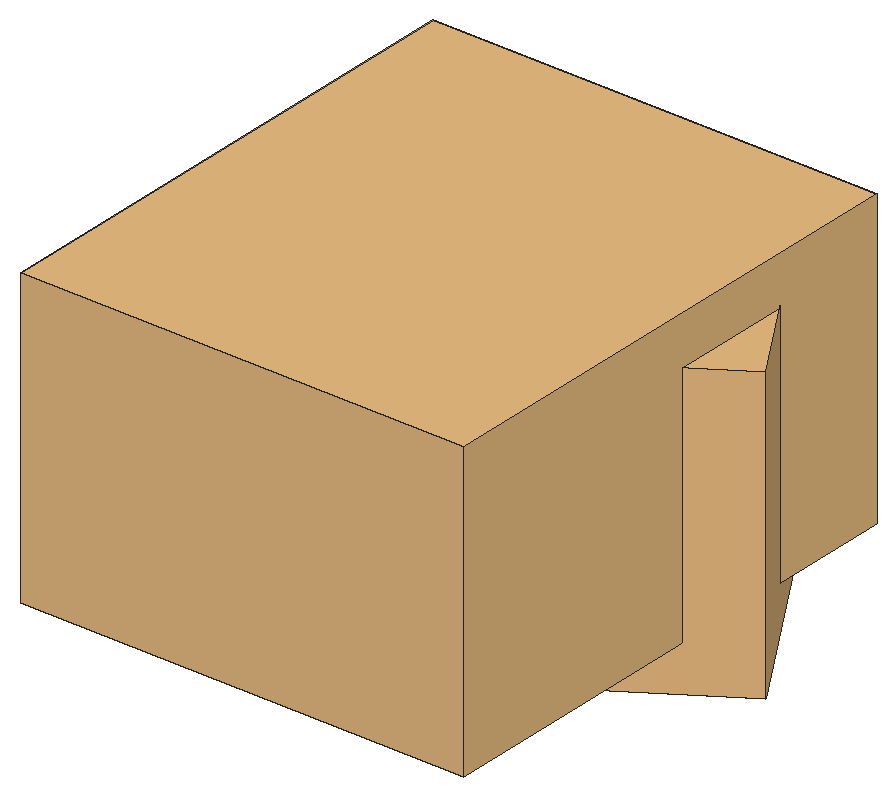
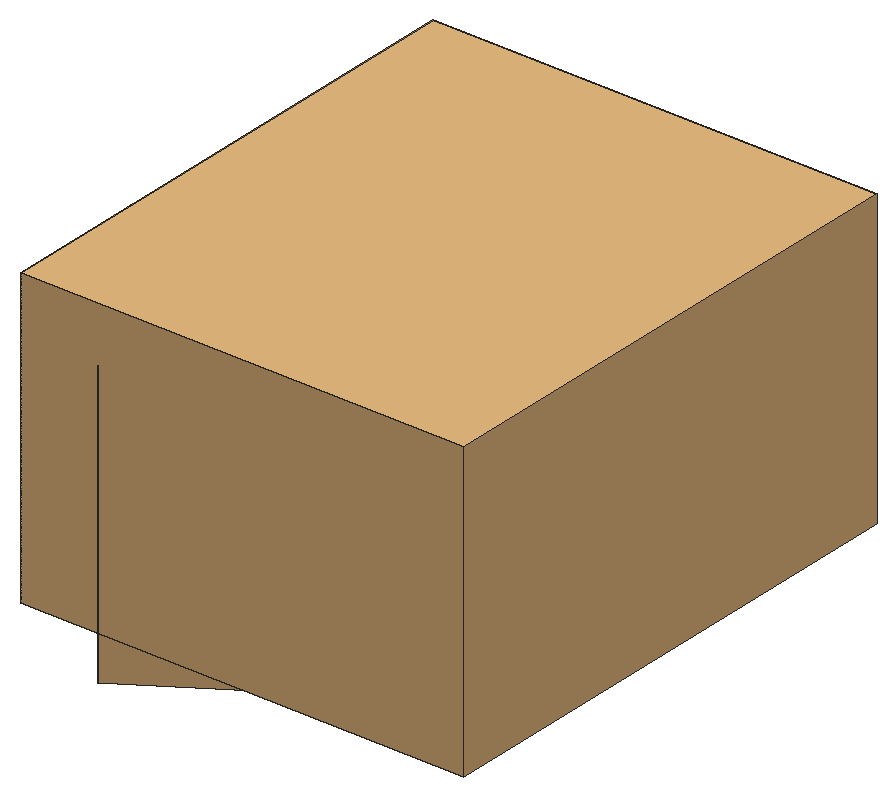
# SketchUp Ruby script. Lengths in inches.
U = 1.inch
M = Sketchup.active_model
def pt(a) = Geom::Point3d.new(a.map { |v| v * U })
def face(e, loops, mat)
  f = e.add_face(loops[0].map { |a| pt(a) })
  loops[1..].each { |l| e.add_face(l.map { |a| pt(a) }).erase! }
  f.material = f.back_material = mat if mat
  f
end
# faces: each face lists its corners as indices into pts; further lists are holes
def faces(e, pts, list, mat = nil) = list.each { |f| face(e, (f[0].is_a?(Array) ? f : [f]).map { |l| l.map { |i| pts[i] } }, mat) }
# xy, xz, yz: faces in a plane at the given z, y or x. An outline is a flat list of corners, or four numbers for a rectangle; further outlines are holes
def ring(l) = l.size == 4 ? [[l[0], l[1]], [l[2], l[1]], [l[2], l[3]], [l[0], l[3]]] : l.each_slice(2).to_a
def flat(e, list, mat, &to3) = list.each { |f| face(e, (f[0].is_a?(Array) ? f : [f]).map { |l| ring(l).map { |u, v| to3.(u, v) } }, mat) }
def xy(e, z, list, mat = nil) = flat(e, list, mat) { |x, y| [x, y, z] }
def xz(e, y, list, mat = nil) = flat(e, list, mat) { |x, z| [x, y, z] }
def yz(e, x, list, mat = nil) = flat(e, list, mat) { |y, z| [x, y, z] }
def lines(e, pts, list) = list.each { |a, b| e.add_line(pt(pts[a]), pt(pts[b])) }
# prism: a flat outline (further loops are holes) pulled along v
def prism(e, loops, v, mat = nil)
  f = face(e, loops, mat); d = Geom::Vector3d.new(v.map { |x| x * U })
  f.pushpull(f.normal.samedirection?(d) ? d.length : -d.length)
end
def box(e, o, s, mat = nil) = prism(e, [[o, [o[0] + s[0], o[1], o[2]], [o[0] + s[0], o[1] + s[1], o[2]], [o[0], o[1] + s[1], o[2]]]], [0, 0, s[2]], mat)
def at(x, y, z, deg = 0) = Geom::Transformation.translation(pt([x, y, z])) * Geom::Transformation.rotation(ORIGIN, Z_AXIS, deg.degrees)
def axes(o, x, y, z) = Geom::Transformation.new([*x, 0, *y, 0, *z, 0, *pt(o).to_a, 1])
def part(name) = M.definitions.add(name)
# library, detail: a bought-in or finely detailed component or shape, given as its bounding box
def library(name, o, s) = part(name).tap { |d| box(d.entities, o, s) }
def detail(e, o, s) = box(e.add_group.entities, o, s)
def put(e, d, t, mat = nil) = e.add_instance(d, t).tap { |i| i.material = mat if mat }
def group(e, t, mat = nil) = e.add_group.tap { |g| g.transformation = t; g.material = mat if mat }.entities
root = M.entities
M.materials.add("0ad16as01f6asdLeafVar1sfd015as60f1as6").color = [231, 235, 211]
M.materials.add("asdfasdf0165f6asdLeafVar1sfd015as60f1as6").color = [231, 235, 211]
M.materials.add("dw_stemssadfasdfa0sdf1s01d6w1").color = [90, 97, 50]
M.materials.add("viburnumblaasdfas0df1w06d").color = [98, 102, 84]
M.materials.add("viburnumbladsadfasdfad0w122").color = [125, 129, 119]
c1 = part("Component\#315")
p = [[0.25,0,0],[2.05,0.01,0.35],[1.81,4.2,1.66],[0,4.19,1.3125]]
faces(c1.entities,p,[[0,1,2,3]],"viburnumbladsadfasdfad0w122")
c2 = part("viburnumblad2")
put(c2.entities,c1,axes([-19.23,-4.49,-32.18],[83.35428,0,0],[0,79.38502,0],[0,0,83.35428]))
c3 = part("Component\#314")
p = [[0.14,0,0],[2.58,0.05,0.25],[2.44,5.11,2.64],[0,5.05,2.39]]
faces(c3.entities,p,[[0,1,2,3]],"viburnumblaasdfas0df1w06d")
c4 = part("viburnumblad1\#2")
put(c4.entities,c3,axes([-37.25,6.23,19.31],[75.98784,0,0],[0,65.50676,0],[0,0,75.98784]))
c5 = part("vdw_leaf\#1")
p = [[0,0,0],[-2.77,1.61,2.32],[-4.3125,6.1,4.5],[-3.97,13.49,6.09],[-2.47,18.57,6.3],[-0.2,22.73,5.75],
  [2.54,19.66,6.85],[4.3,15.93,7.09],[5.03,7.6,5.43],[3.32,1.76,2.74]]
faces(c5.entities,p,[[0,1,2,3,4,5],[0,5,6,7,8,9]],"0ad16as01f6asdLeafVar1sfd015as60f1as6")
c6 = part("dw_branch_3\#2")
p = [[-10.06,-1.6,62.9],[-0.2,1.54,-0.01],[-10.43,1.54,62.72],[0.18,-1.6,0.17],[-23.75,-21.66,88.91],[-25.7,-20.3,89.55],
  [13.4,11.62,104.56],[13.33,13.52,104.47],[-49.25,-41.87,130.3125],[-50.33,-40.21,130.71],[-4.97,21.13,143.98],[35.61,27.99,178.64],
  [-5.09,23.64,143.96],[35.32,29.14,178.46],[-67.7,-55.38,181.06],[-68.34,-54.45,181.62],[-22.8125,33.9,200.59],[-22.94,35.79,200.41],
  [56.61,36.78,229.75],[56.29,38.09,229.57],[-70.63,-67.46,248.85],[-70.72,-66.33,249.5],[-25.05,43.32,240.75],[-24.98,44.26,240.57]]
faces(c6.entities,p,[[0,1,2],[0,3,1],[4,2,5],[4,0,2],[6,0,2],[6,2,7],[8,4,5],[8,5,9],
  [10,6,7],[11,6,7],[10,7,12],[11,7,13],[14,8,9],[14,9,15],[16,10,12],[16,12,17],
  [18,11,13],[18,13,19],[20,14,15],[20,15,21],[22,16,17],[22,17,23]],"dw_stemssadfasdfa0sdf1s01d6w1")
c7 = part("dw_branch3\#2")
put(c7.entities,c5,axes([-70.33,-63.58,233.32],[-1.00752,0.412,0.78596],[-0.24851,-1.22189,0.32195],[0.83141,0.09817,1.01433]))
put(c7.entities,c5,axes([-66.93,-54.91,182.82],[-0.84976,-0.98359,0.33619],[0.99572,-0.74889,0.32577],[-0.05223,0.46521,1.22907]))
put(c7.entities,c5,axes([-46.12,-39.49,126.35],[1.23843,0.5364,0.23552],[-0.56438,0.94474,0.81599],[0.15707,-0.83465,1.07498]))
put(c7.entities,c5,axes([13.0625,13.13,104.77],[-1.01271,0.69982,-0.26884],[-0.74268,-0.99813,0.19939],[-0.10222,0.31872,1.21473]))
put(c7.entities,c5,axes([-18.87,30.42,186.42],[0.36309,1.06515,-0.56675],[-1.14134,0.49515,0.19939],[0.39128,0.45593,1.10754]))
put(c7.entities,c5,axes([-3.2,4.15,75.77],[-1.04153,0.55414,0.44243],[-0.23365,-1.01045,0.71554],[0.6695,0.50943,0.93801]))
put(c7.entities,c5,axes([23.2,19.41,136.3],[-0.65687,-1.11295,-0.05714],[1.05857,-0.61429,-0.20411],[0.15163,-0.1536,1.24868]))
put(c7.entities,c5,axes([-25.57,35.48,201.32],[-0.64726,0.62827,0.87973],[-0.71635,-1.0172,0.19939],[0.80962,-0.39773,0.87973]))
put(c7.entities,c5,axes([-36.37,-32.14,110.35],[-0.80747,1.09962,0.12544],[-0.83333,-0.50188,-0.96467],[-0.72833,-0.64487,0.96467]))
put(c7.entities,c5,axes([-9.89,26.72,156.79],[0.45529,1.02969,0.56572],[-1.16919,0.33753,0.32662],[0.11537,-0.64297,1.07744]))
put(c7.entities,c5,axes([-26.57,46.1,241.0625],[0.00015,0.80921,0.22536],[-0.83985,0.00446,-0.01542],[-0.01605,-0.22532,0.80906]))
put(c7.entities,c5,axes([-9.2,-2.58,61.06],[-1.10001,-0.40312,0.39014],[0.40883,-1.1116,0.00411],[0.35732,0.13566,1.14763]))
put(c7.entities,c5,axes([-69.91,-63.11,233.93],[1.36249,-0.1432,0],[0.13201,1.25603,0.5309],[-0.05549,-0.52799,1.26295]))
put(c7.entities,c5,axes([32.2,25.46,166.13],[0.06878,-1.29051,-0.05714],[1.22165,0.07415,-0.20411],[0.2113,-0.04403,1.24868]))
put(c7.entities,c5,axes([-5.68,-0.66,44.43],[-0.48448,-1.12287,0.17078],[0.98138,-0.33653,0.57135],[-0.48308,0.36756,1.04626]))
put(c7.entities,c5,axes([43.45,32.81,198.64],[0.5408,1.19584,0.14106],[-0.94242,0.32409,0.86557],[0.74952,-0.45533,0.98656]))
put(c7.entities,c5,axes([12.52,14.14,104.98],[1.02694,0.54888,0.41092],[-0.53566,1.05407,-0.06927],[-0.38969,-0.12321,1.13846]))
put(c7.entities,c5,axes([44.55,32.375,198.73],[-0.65687,-1.11295,-0.05714],[1.05857,-0.61429,-0.20411],[0.15163,-0.1536,1.24868]))
put(c7.entities,c5,axes([-5.67,21.17,141.44],[-1.10726,0.43603,-0.32953],[-0.49537,-1.03435,0.29588],[-0.17521,0.40597,1.12589]))
put(c7.entities,c5,axes([55.69,37.84,229.48],[0.18984,0.96334,0.18958],[-0.71996,0.0053,0.69399],[0.66755,-0.26823,0.69457]))
put(c7.entities,c5,axes([-21.52,36.85,205.2],[0.72606,-0.98817,0.14519],[0.94364,0.7084,0.10251],[-0.16885,0.05176,1.19664]))
put(c7.entities,c5,axes([-68.51,-56.35,196.07],[1.16319,0.72381,0],[-0.66725,1.0723,0.5309],[0.28049,-0.45075,1.26295]))
put(c7.entities,c6,at(0.01,-0.09,-0.02),"dw_stemssadfasdfa0sdf1s01d6w1")
put(c7.entities,c5,axes([-2.49,5.18,75.91],[0.78614,-0.90346,-0.30078],[0.86953,0.79562,-0.11715],[0.28546,-0.14014,1.16705]))
put(c7.entities,c5,axes([-23.125,-16.22,82.25],[0.32175,1.32576,0.12544],[-1.33153,0.31835,0.05068],[0.01989,-0.13382,1.3633]))
put(c7.entities,c5,axes([-23.75,41.99,230.3],[0.85958,-0.87451,0.14519],[0.66531,0.75721,0.62192],[-0.54076,-0.36226,1.01955]))
put(c7.entities,c5,axes([27.07,22.48,149.34],[0.92952,-0.64745,-0.62467],[0.50188,1.074,-0.36637],[0.71693,0.02135,1.04468]))
put(c7.entities,c5,axes([17.66,16.25,119.93],[-0.91649,0.83891,-0.3601],[-0.87434,-0.77966,0.40896],[0.0492,0.54447,1.14321]))
put(c7.entities,c5,axes([-68.37,-54.54,181.63],[0.32047,1.28399,0.35434],[-1.33153,0.31835,0.05068],[-0.03484,-0.35624,1.32241]))
put(c7.entities,c5,axes([-28.98,-27.1,96.48],[-0.8814,-0.35966,-0.98523],[0.75246,-1.11336,-0.26672],[-0.73065,-0.71272,0.91382]))
put(c7.entities,c5,axes([-15.23,28.43,172.72],[-1.21149,0.11898,0.32517],[-0.09739,-1.25259,0.09551],[0.33228,0.0667,1.21356]))
put(c7.entities,c5,axes([-17.5625,31.23,186.85],[-0.49275,-1.12287,0.14519],[0.95014,-0.33653,0.62192],[-0.53717,0.36756,1.01955]))
put(c7.entities,c5,axes([26.7,21.22,149.39],[-1.00104,0.22334,0.83093],[0.36894,-1.0402,0.72406],[0.77731,0.78134,0.72643]))
put(c7.entities,c5,axes([-31.125,-24.87,97.38],[0.75482,-0.86936,0.69068],[-0.00159,0.80023,1.00899],[-1.08766,-0.58016,0.45842]))
put(c7.entities,c5,axes([-71.21,-66.73,248.67],[0.25207,0.96771,0],[-0.8921,0.23237,0.38752],[0.375,-0.09768,0.92186]))
put(c7.entities,c5,axes([-24.11,41.05,229.55],[-1.11612,0.51924,-0.26884],[-0.56394,-1.10897,0.19939],[-0.15444,0.29694,1.21473]))
put(c7.entities,c5,axes([6.75,8.37,91.63],[-0.33418,-1.12287,0.39014],[1.13558,-0.33653,0.00411],[0.10478,0.36756,1.14763]))
put(c7.entities,c5,axes([-26,45.89,241.63],[-0.26986,-0.70824,-0.32129],[0.56818,-0.39091,0.38449],[-0.49365,-0.09775,0.63011]))
put(c7.entities,c5,axes([3.74,17.32,124.35],[0.22441,1.22913,-0.16274],[-1.07812,0.11178,-0.64246],[-0.61228,0.25367,1.07162]))
put(c7.entities,c5,axes([-5.44,22.27,140.88],[1.2203,0.00475,0.31374],[-0.097,1.20386,0.35905],[-0.29841,-0.37189,1.1663]))
put(c7.entities,c5,axes([-13.79,29.35,173.31],[0.83169,-0.90108,0.14519],[0.68877,0.73594,0.62192],[-0.55187,-0.34509,1.01955]))
put(c7.entities,c5,axes([-16.92,-7.26,72.98],[1.30647,0.30378,-0.27886],[0.07026,0.74892,1.14503],[0.40633,-1.10623,0.69861]))
put(c7.entities,c5,axes([4.8,17.55,125.22],[-0.25598,-1.17842,0.26559],[1.01553,-0.08455,0.60363],[-0.56975,0.35087,1.00767]))
put(c7.entities,c5,axes([5.3125,8.35,91.45],[0.00638,1.22913,-0.27714],[-1.16413,0.11178,0.46895],[0.48205,0.25367,1.13617]))
put(c7.entities,c5,axes([38.12,30.57,183.07],[1.12534,0.26182,-0.63833],[-0.46674,1.18829,-0.33545],[0.5081,0.51169,1.10563]))
put(c7.entities,c5,axes([-70.41,-60.38,214.47],[-0.41425,1.30587,0],[-1.20383,-0.38188,0.5309],[0.50605,0.16053,1.26295]))
put(c7.entities,c5,axes([37.03,28.75,180.67],[-1.12533,0.00102,-0.63799],[-0.00113,-1.2408,0],[-0.62497,0.00057,1.10237]))
put(c7.entities,c5,axes([30.71,25.35,165.96],[-0.1364,1.29314,0.22715],[-1.08768,-0.23921,0.70862],[0.73536,-0.11394,1.09026]))
put(c7.entities,c5,axes([-38.05,-30.84,110.67],[-0.31533,-1.27379,-0.2839],[1.018,-0.40311,0.67794],[-0.74394,-0.05723,1.08307]))
put(c7.entities,c5,axes([50.11,34.45,213.36],[-1.05669,0.74401,-0.05714],[-0.616,-0.82138,0.69675],[0.37221,0.60904,1.04705]))
put(c7.entities,c5,axes([-65.32,-58.78,200.07],[-1.14597,-0.19668,-0.6713],[0.21784,-1.26924,0],[-0.64812,-0.11124,1.139]))
put(c7.entities,c5,axes([-53.2,-43.37,143.59],[-0.72817,-1.09167,-0.2839],[0.82127,-0.72411,0.67794],[-0.71934,0.19815,1.08307]))
put(c7.entities,c5,axes([-61.1,-50.25,163.67],[-0.52887,1.19686,-0.30066],[-1.10762,-0.57104,-0.32484],[-0.42634,0.12264,1.23812]))
put(c7.entities,c5,axes([-54.12,-42.96,142.67],[0.32175,1.32576,0.12544],[-1.33153,0.31835,0.05068],[0.01989,-0.13382,1.3633]))
put(c7.entities,c5,axes([22.03,20.08,132.3],[1.17066,0.5058,-0.34078],[-0.35758,1.16671,0.50333],[0.49407,-0.35407,1.17172]))
put(c7.entities,c5,axes([-8.59,26.04,158.21],[-0.49275,-1.12287,0.14519],[0.95014,-0.33653,0.62192],[-0.53717,0.36756,1.01955]))
put(c7.entities,c5,axes([49.92,34.03,213.7],[1.24742,-0.35176,0.25024],[0.42127,1.159,-0.4708],[-0.09426,0.52477,1.20753]))
put(c7.entities,c5,axes([-70.34,-67.02,249.05],[-0.57048,-0.79684,0],[0.73827,-0.52855,0.24329],[-0.20203,0.14464,0.92729]))
put(c7.entities,c5,axes([56.04,36.81,228.63],[0.33451,-0.90845,-0.15237],[0.87636,0.33365,-0.06538],[0.11487,-0.11636,0.94597]))
put(c7.entities,c5,axes([-69.93,-60.58,214.88],[-0.45293,-0.99272,-0.78227],[1.14635,-0.58199,0.07483],[-0.40282,-0.65636,1.06615]))
put(c7.entities,c5,axes([-16.77,-8.59,72.7],[-1.22785,0.11509,0.53076],[-0.24879,-1.22495,-0.30991],[0.46742,-0.38989,1.16587]))
put(c7.entities,c5,axes([18.29,17.18,119.24],[1.19981,-0.45946,0.3029],[0.40159,1.22775,0.27158],[-0.37626,-0.1547,1.25575]))
put(c7.entities,c5,axes([-6.73,-0.68,43.74],[0.05346,1.22913,-0.27201],[-1.22696,0.11178,0.26396],[0.28163,0.25367,1.20164]))
put(c7.entities,c5,axes([-58.57,-48.42,160.98],[0.43385,-1.23789,0.39533],[1.04879,0.57965,0.66404],[-0.76727,0.09236,1.13122]))
put(c7.entities,c5,axes([-23.4,38.49,215.38],[0.06762,1.22913,-0.26884],[-1.23909,0.11178,0.19939],[0.21835,0.25367,1.21473]))
put(c7.entities,c5,axes([-22.21,-16.62,83.17],[-0.72817,-1.09167,-0.2839],[0.82127,-0.72411,0.67794],[-0.71934,0.19815,1.08307]))
put(c7.entities,c5,axes([-45.7,-40.77,126.53],[-1.33715,-0.0713,-0.0976],[0.07167,-1.28508,-0.04314],[-0.09306,-0.0492,1.31098]))
put(c7.entities,c5,axes([-22.39,38.51,216.12],[-0.49275,-1.12287,0.14519],[0.95014,-0.33653,0.62192],[-0.53717,0.36756,1.01955]))
c8 = part("vdw_leaf\#2")
p = [[0,0,0],[-2.77,1.61,2.32],[-4.3125,6.1,4.5],[-3.97,13.49,6.09],[-2.47,18.57,6.3],[-0.2,22.73,5.75],
  [2.54,19.66,6.85],[4.3,15.93,7.09],[5.03,7.6,5.43],[3.32,1.76,2.74]]
faces(c8.entities,p,[[0,1,2,3,4,5],[0,5,6,7,8,9]],"asdfasdf0165f6asdLeafVar1sfd015as60f1as6")
c9 = part("dg_branch_1\#2")
p = [[46.12,1.57,35.62],[46,5.42,35.41],[0.14,1.79,0.05],[0.26,-2.0625,0.27],[74.05,2.99,75.8],[74.11,5.28,75.58],
  [103.46,0.47,94.74],[104.03,2.92,94.84],[81.14,16.92,120.46],[81.2,18.78,120.24],[130.47,-5.6875,130.27],[130.58,-3.66,129.85],
  [80.82,34.4375,191.22],[80.64,35.93,190.9],[148.49,-14.56,203.24],[148.9,-12.8125,203.11],[81.08,37.95,226.93],[81.4,39.1,227.03],
  [157.45,-18.19,250.77],[157.7,-17.01,250.41]]
faces(c9.entities,p,[[0,1,2,3],[4,0,1],[4,1,5],[6,4,5],[6,5,7],[8,4,5],[8,5,9],[10,6,7],
  [10,7,11],[12,8,9],[12,9,13],[14,10,11],[14,11,15],[16,12,13],[16,13,17],[18,14,15],
  [18,15,19]],"dw_stemssadfasdfa0sdf1s01d6w1")
c10 = part("vdw_branch1\#3")
put(c10.entities,c8,axes([120.69,-2.42,117.31],[1.12221,-0.24063,-0.65809],[0.19207,1.24776,-0.12871],[0.65778,0.01392,1.11658]))
put(c10.entities,c8,axes([81,38.9,226.05],[0.7888,-0.58155,0],[0.48308,0.65523,0.47],[-0.28484,-0.38635,0.83138]))
put(c10.entities,c8,axes([78.08,12.69,106.05],[-1.43826,-0.02353,-0.03177],[0.0088,-1.31777,0.57755],[-0.03854,0.57714,1.31741]))
put(c10.entities,c8,axes([130.18,-4.73,130.41],[-0.38031,-1.29044,-0.11242],[1.20662,-0.31032,-0.51987],[0.47109,-0.24694,1.24081]))
put(c10.entities,c8,axes([157.08,-17.89,249.93],[-0.91355,0.40674,0],[-0.37496,-0.84216,0.38752],[0.15762,0.35401,0.92186]))
put(c10.entities,c8,axes([90.64,3.03,86.49],[0.32514,-0.85045,-0.99675],[0.69523,0.98247,-0.61148],[1.11061,-0.36604,0.67459]))
put(c10.entities,c8,axes([80.15,28.42,160.95],[-0.16039,0.95636,-1.06292],[-1.41646,0.03966,0.24943],[0.19509,1.07422,0.93709]))
put(c10.entities,c8,axes([126.74,-5.45,129.22],[-0.59819,0.96152,-0.6841],[-0.85772,0.12575,0.92675],[0.75427,0.88089,0.57856]))
put(c10.entities,c8,axes([133.22,-6.12,150.66],[-0.93823,0.76985,0.59124],[-0.47726,-1.08188,0.65135],[0.84525,0.24366,1.02405]))
put(c10.entities,c8,axes([80.43,22.89,141.32],[-1.42571,-0.19312,0.01373],[0.18338,-1.31425,0.5561],[-0.0621,0.5528,1.32692]))
put(c10.entities,c8,axes([33.14,0.88,26.42],[-0.13338,1.31536,0.04876],[-1.04528,-0.13221,0.7073],[0.72315,0.03348,1.07497]))
put(c10.entities,c8,axes([152.63,-15.08,221.76],[-1.28188,0.41945,0.0579],[-0.3638,-1.18547,0.53367],[0.21665,0.49113,1.23869]))
put(c10.entities,c8,axes([80.05,28.28,160.33],[-0.46732,-1.26661,0.40679],[1.27397,-0.40257,0.21004],[-0.07408,0.44645,1.30501]))
put(c10.entities,c8,axes([153.95,-14.8,235.875],[0.39005,1.07743,0.20605],[-0.96443,0.25296,0.50293],[0.42961,-0.3464,0.99807]))
put(c10.entities,c8,axes([80.2,24.22,141.74],[1.33062,-0.46576,0.02628],[0.44746,1.2746,-0.06608],[-0.00197,0.0722,1.37936]))
put(c10.entities,c8,axes([145.48,-12.5,188.92],[-1.32952,0.16983,0.16138],[-0.09299,-1.2361,0.53471],[0.21503,0.51548,1.22904]))
put(c10.entities,c8,axes([139.64,-9.18,171.24],[0.05682,1.30088,0.23414],[-1.13176,-0.05343,0.57151],[0.58357,-0.22963,1.13417]))
put(c10.entities,c8,axes([70.95,4.35,71.98],[-1.1081,-0.41873,0.64752],[0.33675,-1.28259,-0.25313],[0.6937,-0.04625,1.15721]))
put(c10.entities,c8,axes([59.85,4.55,56.17],[-0.26797,1.24526,0.35754],[-0.9369,-0.41634,0.74783],[0.83377,-0.10389,0.98674]))
put(c10.entities,c8,axes([33.11,3.36,25.66],[-0.57817,-1.07968,-0.5679],[1.11554,-0.21356,-0.7297],[0.49375,-0.78178,0.98363]))
put(c10.entities,c9,at(-0.21,0.34,-0.17),"dw_stemssadfasdfa0sdf1s01d6w1")
put(c10.entities,c8,axes([80.91,19.01,122.53],[-0.84258,1.13222,-0.27981],[-1.15093,-0.75138,0.42537],[0.18861,0.47293,1.3457]))
put(c10.entities,c8,axes([119.8,-1.22,114.1],[-1.3235,-0.25012,0.09101],[0.25933,-1.31572,0.15537],[0.05991,0.1698,1.33794]))
put(c10.entities,c8,axes([46.29,5.1,38.04],[0.98937,0.73827,-0.47585],[-0.72359,1.03721,0.10473],[0.44068,0.18581,1.20453]))
put(c10.entities,c8,axes([81.1875,33.03,184.45],[1.33883,0.26986,0.35053],[-0.09581,1.22087,-0.57399],[-0.42216,0.53228,1.20262]))
put(c10.entities,c8,axes([80.16,36.28,206.98],[-0.83993,0.85737,-0.6234],[-1.05964,-0.65701,0.5241],[0.02941,0.81391,1.07976]))
put(c10.entities,c8,axes([154.86,-16.15,234.87],[0.02509,-1.15302,-0.28506],[1.1487,-0.04894,0.29908],[-0.30202,-0.28195,1.11384]))
put(c10.entities,c8,axes([108.77,-0.33,101.14],[-0.47691,-1.03266,-0.72709],[1.25395,-0.29455,-0.40416],[0.15052,-0.81814,1.06325]))
put(c10.entities,c8,axes([89.79,3.01,85.87],[-0.61344,0.75518,0.8965],[-0.17758,-1.01824,0.73622],[1.13385,0.22574,0.58569]))
put(c10.entities,c8,axes([81.56,20.31,123.29],[0.37259,-1.3435,0.21057],[1.29385,0.32364,-0.22445],[0.16906,0.25791,1.34638]))
put(c10.entities,c8,axes([46.45,1.82,36.74],[-0.77883,0.29892,1.0614],[0.19124,-1.24314,0.49044],[1.08598,0.43329,0.67484]))
put(c10.entities,c8,axes([71.37,4.02,72.32],[0.72905,0.81546,-0.74421],[-0.66805,0.98958,0.42988],[0.8391,0.14186,0.97745]))
put(c10.entities,c8,axes([136.59,-5.88,150.53],[0.85845,-0.99897,-0.12437],[0.96526,0.81273,0.13453],[-0.02572,-0.18182,1.28292]))
put(c10.entities,c8,axes([80.375,38.8,225.86],[-0.25178,0.96778,0],[-0.89216,-0.23211,0.38752],[0.37503,0.09757,0.92186]))
put(c10.entities,c8,axes([74.43,7.99,85.38],[-1.05703,0.91669,-0.33543],[-0.95806,-0.87958,0.61531],[0.18697,0.6754,1.25659]))
put(c10.entities,c8,axes([76.57,9.74,89.32],[0.63146,-1.21538,0.33508],[1.18148,0.49387,-0.43517],[0.26321,0.48577,1.26593]))
put(c10.entities,c8,axes([81.6875,36.97,207.4],[0.09422,-1.04424,0.38486],[1.01646,0.1939,0.27727],[-0.33299,0.33382,0.98727]))
put(c10.entities,c8,axes([157.29,-17.17,249.98],[0.50586,-0.50586,0],[0.38853,0.38853,0.41105],[-0.29684,-0.29684,0.56115]))
put(c10.entities,c8,axes([79.92,15.8,106.09],[1.03917,-0.29343,-0.90675],[-0.14587,1.22131,-0.5624],[0.92163,0.5191,0.88824]))
put(c10.entities,c8,axes([61.95,3.88,56.26],[0.41243,-1.28546,0],[1.17466,0.37688,-0.54831],[0.5221,0.16751,1.23363]))
put(c10.entities,c8,axes([151.99,-14.79,208.15],[-0.48571,-1.21723,-0.32393],[1.25386,-0.50033,0],[-0.12005,-0.30087,1.31056]))
put(c10.entities,c8,axes([108.44,0.62,102.22],[0.82183,0.96078,0.38967],[-0.62327,0.08618,1.10203],[0.79141,-0.88661,0.51693]))
put(c10.entities,c8,axes([145.6,-10.56,188.62],[1.03241,-0.02554,-0.82693],[0.3944,1.11584,0.45794],[0.70325,-0.61672,0.89706]))
put(c10.entities,c8,axes([78.59,32.3,183.89],[-1.12675,-0.42036,0.43987],[0.5899,-0.98149,0.57312],[0.14901,0.70693,1.05726]))
put(c10.entities,c8,axes([152.08,-13.42,223.37],[0.79993,-0.44251,-0.69938],[0.68456,0.82615,0.26026],[0.41048,-0.60953,0.85515]))
put(c10.entities,c8,axes([140.71,-8.74,170.55],[0.41903,-1.24177,-0.32393],[1.26224,0.33728,0.33986],[-0.23168,-0.40836,1.26573]))
put(c10.entities,c8,axes([149.25,-12.53,205.78],[1.24456,0.38285,0.23414],[-0.42999,1.04826,0.57151],[-0.02056,-0.62679,1.13417]))
c11 = part("vdw_leaf\#3")
p = [[0,0,0],[-2.77,1.61,2.32],[-4.3125,6.1,4.5],[-3.97,13.49,6.09],[-2.47,18.57,6.3],[-0.2,22.73,5.75],
  [2.54,19.66,6.85],[4.3,15.93,7.09],[5.03,7.6,5.43],[3.32,1.76,2.74]]
faces(c11.entities,p,[[0,1,2,3,4,5],[0,5,6,7,8,9]],"asdfasdf0165f6asdLeafVar1sfd015as60f1as6")
c12 = part("dw_brancj_2\#2")
p = [[9.7,-0.22,29.95],[0.23,-1.96,0.34],[-0.05,1.51,0.11],[9.65,1.51,29.46],[18.64,-8.75,84.43],[18.96,-6.63,84.625],
  [1.53,6.02,63.68],[1.42,8.18,63.25],[-10.58,8.77,161.17],[-10.41,9.98,160.68],[26.34,-9.37,211.72],[26.57,-8.28,211.23]]
faces(c12.entities,p,[[0,1,2],[0,2,3],[4,0,3],[4,3,5],[6,0,3],[6,3,7],[8,6,7],[8,7,9],
  [10,4,5],[10,5,11]],"dw_stemssadfasdfa0sdf1s01d6w1")
c13 = part("vdw_branch2\#3")
put(c13.entities,c11,axes([19.53,-5.9,102.42],[1.12377,-0.50004,0],[0.46097,1.03596,0.47664],[-0.19377,-0.43548,1.13389]))
put(c13.entities,c11,axes([-5.89,6.52,109.44],[-1.07209,0.83679,0],[-0.77141,-0.98832,0.52702],[0.32427,0.41545,1.25373]))
put(c13.entities,c11,axes([-0.44,8.23,75.28],[0.88709,-0.9947,0],[0.92159,0.82189,0.33087],[-0.25219,-0.22491,1.26111]))
put(c13.entities,c11,axes([24.71,-8.97,190.81],[-0.82641,0.91101,0],[-0.83983,-0.76184,0.47664],[0.35303,0.32025,1.13389]))
put(c13.entities,c11,axes([-2.29,8.24,91.35],[1.24603,-0.47303,0],[0.43826,1.15445,0.33087],[-0.11993,-0.31592,1.26111]))
put(c13.entities,c11,axes([12.26,-3.11,37.92],[-0.64625,1.02205,0.22511],[-1.04383,-0.61044,-0.22511],[-0.07533,-0.30931,1.18809]))
put(c13.entities,c11,axes([26.17,-9.17,210.27],[-0.99452,-0.10453,0],[0.09636,-0.91681,0.38752],[-0.04051,0.38539,0.92186]))
put(c13.entities,c11,axes([-6.07,9.4,125.35],[-0.90214,-0.98107,0],[0.90896,-0.83583,0.33087],[-0.24874,0.22873,1.26111]))
put(c13.entities,c11,axes([-4.13,7.29,110.58],[0.44715,-1.078,0.64369],[1.05816,0.63649,0.33087],[-0.58725,0.40856,1.09216]))
put(c13.entities,c11,axes([23.91,-8.22,171.96],[0.62307,0.85009,-0.63406],[-0.71531,0.8798,0.47664],[0.78296,0.12729,0.94004]))
put(c13.entities,c12,at(-0.09,0.18,-0.25),"dw_stemssadfasdfa0sdf1s01d6w1")
put(c13.entities,c11,axes([23.34,-9.65,156.59],[-0.31364,-1.00782,0.58216],[1.10369,-0.17062,0.29925],[-0.17137,0.6239,0.98776]))
put(c13.entities,c11,axes([15.03,-3.37,58.83],[-1.05425,-0.00194,0.58442],[-0.14303,-1.11707,-0.26172],[0.55355,-0.3046,0.99755]))
put(c13.entities,c11,axes([-11.625,9.46,160.37],[0.36812,0.92978,0],[-0.85713,0.33936,0.38752],[0.3603,-0.14265,0.92186]))
put(c13.entities,c11,axes([21.32,-8.53,138.72],[1.21379,0.19904,0],[-0.19904,1.21379,0],[0,0,1.23]))
put(c13.entities,c11,axes([22.54,-9.2,141.43],[-1.02887,0.17955,0.60182],[-0.23387,-1.13057,-0.06253],[0.56696,-0.17376,1.02111]))
put(c13.entities,c11,axes([23.9,-8.82,173.84],[-1.14567,-0.37474,0],[0.35918,-1.0981,0.04438],[-0.01409,0.04308,1.17993]))
put(c13.entities,c11,axes([-7.84,8.92,143.59],[-1.26971,0.40522,0],[-0.37543,-1.17638,0.33087],[0.10274,0.32192,1.26111]))
put(c13.entities,c11,axes([19.77,-8.01,85.98],[-0.32405,-1.14591,0.18674],[1.10278,-0.32969,-0.10948],[0.15845,0.14442,1.16117]))
put(c13.entities,c11,axes([-0.62,5.76,76.34],[-0.08879,1.17576,-0.67771],[-1.34525,-0.16582,-0.11144],[-0.17897,0.66309,1.17383]))
put(c13.entities,c11,axes([20.49,-8.22,121.07],[0.39924,-0.78471,-0.8233],[1.08735,0.33121,0.2116],[0.09035,-0.83005,0.83495]))
put(c13.entities,c11,axes([15.15,-3.72,62.9],[1.16251,0.40128,-0.0211],[-0.39924,1.16074,0.07874],[0.0456,-0.06757,1.2273]))
put(c13.entities,c11,axes([20.72,-8.08,120.26],[-0.03693,1.2277,-0.06551],[-1.22944,-0.03698,0],[-0.00197,0.06548,1.22825]))
put(c13.entities,c11,axes([22.58,-8.36,155.57],[-0.56247,1.09386,0],[-1.00839,-0.51852,0.47664],[0.42389,0.21796,1.13389]))
put(c13.entities,c11,axes([3.97,3.13,57.96],[-1.09459,0.76041,0],[-0.72262,-1.0402,-0.1735],[-0.10109,-0.14552,1.29352]))
put(c13.entities,c11,axes([-10.8,9.06,160.75],[-0.66334,-0.72138,0],[0.66835,-0.61458,0.24329],[-0.1829,0.16818,0.92729]))
put(c13.entities,c11,axes([19.06,-9.3125,103.96],[-1.01345,0.25553,-0.60051],[-0.2265,-1.12952,-0.09839],[-0.59598,0.03076,1.01889]))
put(c13.entities,c11,axes([18.07,-6.2,81.7],[-0.56247,1.09386,0],[-1.00839,-0.51852,0.47664],[0.42389,0.21796,1.13389]))
put(c13.entities,c11,axes([12.95,-0.39,43.31],[0.13044,-1.19832,0],[1.11025,0.12085,0.29925],[-0.30382,-0.03307,1.14057]))
put(c13.entities,c11,axes([2.28,8.28,56.18],[1.32413,-0.31027,0],[0.30923,1.31968,-0.11144],[0.02542,0.1085,1.35543]))
put(c13.entities,c11,axes([-7.55,9.96,143.07],[1.34251,-0.21744,0],[0.20045,1.23761,0.52702],[-0.08426,-0.52024,1.25373]))
put(c13.entities,c11,axes([26.15,-8.25,210.66],[0.94661,-0.25364,0],[0.235,0.87703,0.24329],[-0.06431,-0.24,0.92729]))
put(c13.entities,c11,axes([-6.48,11.37,125.16],[0.64635,1.10315,0.46356],[-1.16569,0.46153,0.52702],[0.27017,-0.6478,1.16488]))
put(c13.entities,c11,axes([25.74,-8.35,191.28],[0.13044,-1.19832,0],[1.11025,0.12085,0.29925],[-0.30382,-0.03307,1.14057]))
put(c13.entities,c11,axes([-5.125,7.47,91.6],[-1.10024,0.63688,0.48318],[-0.78682,-1.00808,-0.46292],[0.14137,-0.65404,1.184]))
c14 = library("Broadleaf plant",[0,0,0],[62.33,72.62,41.59])
c15 = library("Narrowleaf plant",[-0.44,-0.75,-1.28],[7.48,8.05,9.01])
put(root,c2,axes([2217.49,336.92,16.58],[-0.00784,0.00117,0.00859],[-0.00546,-0.0084,-0.00383],[0.00631,-0.00716,0.00674]))
put(root,c2,axes([2214.78,333.28,28.73],[0.00871,-0.00384,-0.00541],[0.00664,0.00406,0.00749],[-0.00079,-0.00912,0.00457]))
put(root,c2,axes([2214.99,335.42,27.42],[0.00909,-0.00401,-0.00564],[0.00597,0.00365,0.00674],[-0.00079,-0.00912,0.00457]))
put(root,c2,axes([2216.93,338.17,16.16],[-0.01071,-0.0052,0.00268],[0.00135,-0.00683,-0.00788],[0.0054,-0.00736,0.0073]))
put(root,c2,axes([2216.82,342,22.89],[-0.01242,-0.00411,0.00252],[0.00364,-0.01255,-0.00256],[0.00316,-0.0017,0.01283]))
put(root,c2,axes([2215.32,334.5625,28.24],[0.00143,-0.00635,-0.00868],[0.00992,-0.00012,0.00155],[-0.0013,-0.00861,0.00528]))
put(root,c4,axes([2216.48,338.3,27.22],[0.01164,0.00293,-0.00079],[-0.00215,0.01041,0.00877],[0.00216,-0.00738,0.00809]))
put(root,c2,axes([2216.16,333.26,28.67],[-0.00668,-0.00514,-0.00687],[0.00865,-0.00485,-0.0047],[-0.00103,-0.00803,0.00606]))
put(root,c2,axes([2216.17,335.37,27.46],[-0.00601,-0.0039,-0.00689],[0.00865,-0.00485,-0.0047],[-0.00175,-0.00854,0.00529]))
put(root,c4,axes([2216.23,342.42,26.16],[-0.01393,-0.0074,0.00333],[0.00558,-0.01491,-0.00981],[0.00654,-0.00631,0.01332]))
put(root,c4,axes([2215.12,339.45,25.59],[0.00605,-0.00776,-0.00693],[0.01168,0.0029,0.00677],[-0.00267,-0.00844,0.00676]))
put(root,c2,axes([2215.8,343.2,21.68],[-0.0065,-0.01157,-0.00112],[0.01142,-0.00611,-0.00313],[0.00221,-0.00249,0.0129]))
put(root,c4,axes([2215.51,340.6,15.08],[-0.00788,-0.01001,-0.0014],[0.00865,-0.00529,-0.01087],[0.00682,-0.00657,0.00863]))
put(root,c2,axes([2216.59,335.63,18.54],[0.01026,0.00498,-0.00256],[-0.00015,0.00559,0.01026],[0.0056,-0.00897,0.00496]))
put(root,c2,axes([2218.89,346.86,25.88],[-0.00545,0.00916,0.00529],[-0.00808,-0.00821,0.00589],[0.00818,-0.00089,0.00998]))
put(root,c4,axes([2216.46,349.125,21.13],[-0.00936,-0.00465,0.0096],[0.00338,-0.01554,-0.00424],[0.01026,-0.00044,0.00979]))
put(root,c2,axes([2215.58,342.97,23.5],[0.00323,-0.01225,-0.0041],[0.01276,0.00369,-0.00099],[0.00204,-0.00369,0.01263]))
put(root,c2,axes([2217.47,339.64,30.71],[-0.01238,-0.00774,-0.00167],[0.00772,-0.01057,-0.00819],[0.00296,-0.0074,0.01235]))
put(root,c2,axes([2216.15,337.13,18.125],[0.00784,-0.00117,-0.00859],[0.00729,0.00715,0.00568],[0.00468,-0.00917,0.00553]))
put(root,c2,axes([2215.99,338.4375,17.28],[0.00079,-0.00637,-0.0092],[0.01172,0.00425,-0.00193],[0.00425,-0.00877,0.00644]))
put(root,c2,axes([2218.42,336.31,17.8],[-0.01026,-0.00498,0.00256],[0.0015,-0.00759,-0.00876],[0.0054,-0.00736,0.0073]))
put(root,c4,axes([2215.96,340.18,26.33],[0.00918,-0.00623,-0.00469],[0.00881,0.01006,0.00379],[0.00131,-0.00544,0.00952]))
put(root,c4,axes([2216.52,341.22,24.43],[-0.00713,-0.00827,-0.00706],[0.01264,-0.00623,-0.00545],[-0.00006,-0.00799,0.0088]))
put(root,c2,axes([2217.31,337.65,17.73],[-0.00667,-0.00821,-0.00496],[0.00888,-0.00228,-0.00816],[0.00454,-0.00802,0.00718]))
put(root,c2,axes([2216.21,340.92,29.79],[-0.0037,-0.01142,-0.00741],[0.01514,-0.00214,-0.00425],[0.00214,-0.0084,0.01187]))
put(root,c4,axes([2218.31,345,27.22],[0.00679,0.01089,0.00142],[-0.00667,0.00218,0.0129],[0.00902,-0.00665,0.00468]))
put(root,c4,axes([2216.41,341.78,24.47],[-0.00228,-0.0125,-0.00287],[0.01428,-0.00152,-0.00471],[0.00336,-0.00314,0.01093]))
put(root,c2,axes([2220.65,346.2,28.34],[-0.00501,0.0098,0.00679],[-0.00808,-0.00821,0.00589],[0.00877,-0.00196,0.0093]))
put(root,c2,axes([2217.59,336.63,18.98],[0.00083,-0.00664,-0.00958],[0.01085,0.00394,-0.00179],[0.00425,-0.00877,0.00644]))
put(root,c2,axes([2219.35,347.77,16.85],[-0.00779,-0.00011,0.00854],[0.00262,-0.01208,0.00224],[0.0089,0.00345,0.00816]))
put(root,c2,axes([2220.25,347.42,26.83],[-0.00997,0.00134,0.00814],[-0.00176,-0.01174,-0.00023],[0.00802,-0.0014,0.01005]))
put(root,c2,axes([2219.27,348.2,25.85],[-0.00949,-0.00826,0.00492],[0.00532,-0.00908,-0.00498],[0.00706,-0.00173,0.0107]))
put(root,c2,axes([2219.68,337.12,29.75],[-0.0092,-0.00594,0.0008],[0.00497,-0.0084,-0.00522],[0.00323,-0.00386,0.00866]))
put(root,c2,axes([2218.71,338.05,29.3],[-0.00331,-0.00841,-0.00433],[0.01007,-0.00189,-0.00393],[0.00222,-0.00567,0.00805]))
put(root,c2,axes([2221.18,344.42,27.9],[-0.00309,0.00736,0.0079],[-0.00654,-0.00921,0.0057],[0.00929,-0.00262,0.00521]))
put(root,c2,axes([2221.22,347.72,28.35],[-0.00909,-0.00791,0.00471],[0.00591,-0.01009,-0.00553],[0.00706,-0.00173,0.0107]))
put(root,c2,axes([2222.57,344.43,28.43],[-0.00733,-0.00034,0.00907],[-0.00172,-0.01154,-0.00184],[0.00876,-0.00225,0.00608]))
put(root,c2,axes([2222.29,345.56,29.38],[-0.00278,-0.01118,-0.00257],[0.00839,-0.00011,-0.00838],[0.00753,-0.00365,0.00688]))
put(root,c2,axes([2223.71,344.5625,29.41],[-0.00715,-0.00814,0.0046],[0.00423,-0.00805,-0.00746],[0.00803,-0.00268,0.00677]))
put(root,c2,axes([2222.86,344.76,30.59],[0.00322,-0.00766,-0.00823],[0.00813,0.00764,-0.00386],[0.00755,-0.0046,0.00633]))
put(root,c7,axes([2240.19,350.04,3.93],[-0.12304,0.0546,-0.04713],[-0.02701,-0.11428,-0.0937],[-0.06098,-0.05955,0.13659]))
put(root,c10,axes([2237.13,349.65,7.1875],[0.01907,-0.13922,0],[0.13922,0.01907,0],[0,0,0.17291]))
put(root,c13,axes([2239.62,349.57,5.4],[0.09858,-0.0952,-0.10951],[0.11351,0.11754,0],[0.06402,-0.06182,0.16863]))
put(root,c14,axes([2211.5625,273.43,8.57],[1.41,0,0],[0,1.41,0],[0,0,1.41]))
put(root,c10,axes([2276.9375,325.67,2.97],[-0.07583,0.05409,0],[-0.05409,-0.07583,0],[0,0,0.11461]))
put(root,c13,axes([2274.88,324.8,3.23],[-0.06851,-0.04024,-0.04853],[0.04493,-0.07649,0],[-0.03401,-0.01998,0.09777]))
put(root,c13,axes([2274.78,325.72,3.73],[-0.10632,-0.02382,-0.02533],[0.02424,-0.1082,0],[-0.02009,-0.0045,0.13407]))
put(root,c7,axes([2278.89,328.36,5.28],[0.06434,-0.05829,0.02833],[0.05722,0.06809,0.01535],[-0.02555,0.00573,0.10572]))
put(root,c15,axes([2304.91,334.49,7.7],[-3.47843,5.41821,0],[-5.41821,-3.47843,0],[0,0,6.43866]))
put(root,c13,axes([2279.46,327.04,2.375],[0.00659,0.0958,-0.06822],[-0.11062,0.0076,0],[0.0038,0.05531,0.11816]))
put(root,c13,axes([2282.24,324.44,1.88],[0.01852,0.08442,-0.0614],[-0.09748,0.02138,0],[0.01069,0.04874,0.10635]))
put(root,c13,axes([2282.86,323.98,3.73],[0.10716,0.01972,-0.02533],[-0.02007,0.10905,0],[0.02025,0.00373,0.13407]))
put(root,c10,axes([2281.35,324.9375,2.97],[0.07973,0.03352,0],[-0.03352,0.07973,0],[0,0,0.10642]))
